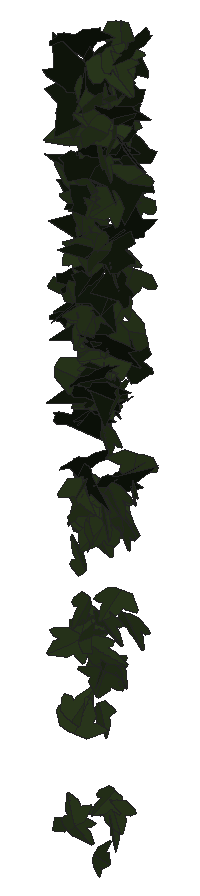
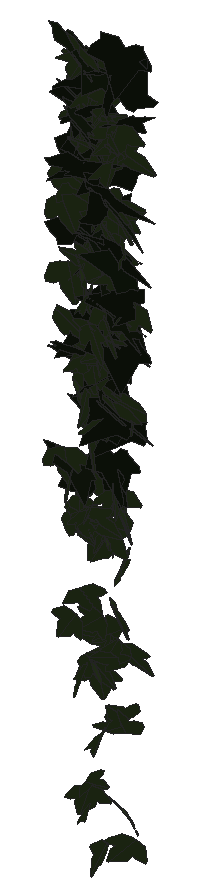
# SketchUp Ruby script. Lengths in inches.
U = 1.inch
M = Sketchup.active_model
def pt(a) = Geom::Point3d.new(a.map { |v| v * U })
def face(e, loops, mat)
  f = e.add_face(loops[0].map { |a| pt(a) })
  loops[1..].each { |l| e.add_face(l.map { |a| pt(a) }).erase! }
  f.material = f.back_material = mat if mat
  f
end
# faces: each face lists its corners as indices into pts; further lists are holes
def faces(e, pts, list, mat = nil) = list.each { |f| face(e, (f[0].is_a?(Array) ? f : [f]).map { |l| l.map { |i| pts[i] } }, mat) }
# xy, xz, yz: faces in a plane at the given z, y or x. An outline is a flat list of corners, or four numbers for a rectangle; further outlines are holes
def ring(l) = l.size == 4 ? [[l[0], l[1]], [l[2], l[1]], [l[2], l[3]], [l[0], l[3]]] : l.each_slice(2).to_a
def flat(e, list, mat, &to3) = list.each { |f| face(e, (f[0].is_a?(Array) ? f : [f]).map { |l| ring(l).map { |u, v| to3.(u, v) } }, mat) }
def xy(e, z, list, mat = nil) = flat(e, list, mat) { |x, y| [x, y, z] }
def xz(e, y, list, mat = nil) = flat(e, list, mat) { |x, z| [x, y, z] }
def yz(e, x, list, mat = nil) = flat(e, list, mat) { |y, z| [x, y, z] }
def lines(e, pts, list) = list.each { |a, b| e.add_line(pt(pts[a]), pt(pts[b])) }
# prism: a flat outline (further loops are holes) pulled along v
def prism(e, loops, v, mat = nil)
  f = face(e, loops, mat); d = Geom::Vector3d.new(v.map { |x| x * U })
  f.pushpull(f.normal.samedirection?(d) ? d.length : -d.length)
end
def box(e, o, s, mat = nil) = prism(e, [[o, [o[0] + s[0], o[1], o[2]], [o[0] + s[0], o[1] + s[1], o[2]], [o[0], o[1] + s[1], o[2]]]], [0, 0, s[2]], mat)
def at(x, y, z, deg = 0) = Geom::Transformation.translation(pt([x, y, z])) * Geom::Transformation.rotation(ORIGIN, Z_AXIS, deg.degrees)
def axes(o, x, y, z) = Geom::Transformation.new([*x, 0, *y, 0, *z, 0, *pt(o).to_a, 1])
def part(name) = M.definitions.add(name)
# library, detail: a bought-in or finely detailed component or shape, given as its bounding box
def library(name, o, s) = part(name).tap { |d| box(d.entities, o, s) }
def detail(e, o, s) = box(e.add_group.entities, o, s)
def put(e, d, t, mat = nil) = e.add_instance(d, t).tap { |i| i.material = mat if mat }
def group(e, t, mat = nil) = e.add_group.tap { |g| g.transformation = t; g.material = mat if mat }.entities
root = M.entities
M.materials.add("1026 AP 7946 SUNNY SIDE UP").color = [254, 231, 186]
M.materials.add("efeu1").color = [18, 25, 13]
M.materials.add("efeu2").color = [43, 57, 29]
c1 = part("ivyleaf_9")
p = [[1.54,2.16,1.25],[1.36,2.04,1.19],[-0.21,0.99,0.68],[-0.71,1.11,0.82],[-0.85,0.86,0.67],[-0.8,0.17,0.21],
  [-0.9,-0.01,0.1],[-0.67,-0.16,-0.02],[-0.08,-0.08,-0.05],[-0.03,-0.6,-0.4],[0.65,-0.88,-0.66],[0.83,-0.6,-0.49],
  [1.29,-0.42,-0.43],[1.8125,-0.07,-0.26],[1.21,0.44,0.15]]
faces(c1.entities,p,[[0,1,2,3,4,5,6,7,8,9,10,11,12,13,14]],"efeu1")
c2 = part("ivyleaf_10")
p = [[0,0.5,-0.03],[-0.0625,2.02,-0.43],[-0.19,2.01,-0.46],[-0.54,1.05,-0.29],[-0.52,0.625,-0.18],[-0.83,0.76,-0.28],
  [-1.16,0.64,-0.33],[-1.15,0.33,-0.24],[-0.77,-0.39,0.02],[-0.3,-0.51,0.16],[0.04,-0.48,0.23],[-0.02,2.01,-0.4375],
  [-0.06,2.01,-0.43],[0.04,-0.49,0.23],[0.67,-0.49,0.14],[1.38,0.36,-0.2],[1.375,0.51,-0.24],[0.81,0.65,-0.19],
  [0.62,0.59,-0.15],[0.6,1.09,-0.28],[0.5,1.23,-0.31]]
faces(c2.entities,p,[[0,1,2,3,4,5,6,7,8,9,10],[11,12,0,13,14,15,16,17,18,19,20]],"efeu2")
put(root,c1,axes([144.33,212.75,264.91],[-0.14477,0.20271,0.14343],[-0.09763,0.12342,-0.22859],[-0.3731,-0.11095,0.00416]),"1026 AP 7946 SUNNY SIDE UP")
put(root,c2,axes([144.375,212.71,265.98],[-0.19313,-0.02932,0.23995],[-0.32391,-0.11299,-0.12713],[0.17757,-0.238,0.02907]),"1026 AP 7946 SUNNY SIDE UP")
put(root,c2,axes([144.0625,212.68,263.17],[-0.37059,0.02772,-0.05912],[0.08531,-0.02917,-0.24359],[-0.05298,-0.24085,0.02125]),"1026 AP 7946 SUNNY SIDE UP")
put(root,c1,axes([144.14,212.86,262.6],[0.23847,0.17879,-0.10822],[-0.08985,-0.09038,-0.24165],[-0.31429,0.1615,-0.01303]),"1026 AP 7946 SUNNY SIDE UP")
put(root,c2,axes([144.39,212.74,264.93],[-0.15157,0.01941,-0.24619],[-0.33509,0.11135,0.09848],[0.17314,0.2325,-0.02493]),"1026 AP 7946 SUNNY SIDE UP")
put(root,c2,axes([143.85,212.85,261.51],[-0.01401,-0.04206,-0.23299],[0.32856,-0.09558,0.00928],[-0.15039,-0.2049,0.04199]),"1026 AP 7946 SUNNY SIDE UP")
put(root,c2,axes([144.24,212.6,256.93],[0.27563,-0.04144,-0.12893],[-0.20017,-0.00058,-0.18384],[0.05252,0.21525,-0.02401]),"1026 AP 7946 SUNNY SIDE UP")
put(root,c1,axes([144.43,212.85,264.24],[-0.08439,-0.01917,-0.25421],[-0.38224,-0.04278,0.05767],[-0.07224,0.24877,-0.00816]),"1026 AP 7946 SUNNY SIDE UP")
put(root,c2,axes([144.13,212.96,261.5],[0.36599,-0.07417,-0.01921],[-0.03604,-0.01206,-0.25102],[0.11456,0.23316,-0.0176]),"1026 AP 7946 SUNNY SIDE UP")
put(root,c2,axes([144.04,212.76,253.56],[-0.25435,-0.06715,-0.11637],[0.17582,0.02264,-0.17929],[0.10757,-0.19578,0.01789]),"1026 AP 7946 SUNNY SIDE UP")
put(root,c1,axes([144.47,212.96,265.19],[-0.2155,0.09765,0.19048],[-0.26082,0.08275,-0.17171],[-0.19892,-0.21428,0.01879]),"1026 AP 7946 SUNNY SIDE UP")
put(root,c1,axes([144.32,212.625,263.04],[-0.13864,0.24377,-0.07114],[0.03024,-0.06794,-0.2674],[-0.39784,-0.09012,0.00447]),"1026 AP 7946 SUNNY SIDE UP")
put(root,c1,axes([144.4,212.91,261.39],[-0.33839,0.1175,-0.00233],[-0.02931,-0.04016,-0.2487],[-0.18248,-0.21145,0.04428]),"1026 AP 7946 SUNNY SIDE UP")
put(root,c2,axes([144.27,212.79,264.34],[-0.28714,0.16387,0.07867],[-0.11276,0.03256,-0.2515],[-0.26028,-0.19488,0.02216]),"1026 AP 7946 SUNNY SIDE UP")
put(root,c2,axes([144.09,212.92,257],[-0.00415,-0.03981,0.2256],[0.07202,0.21445,0.04194],[-0.34285,0.04553,0.00608]),"1026 AP 7946 SUNNY SIDE UP")
put(root,c2,axes([144.19,212.77,259.43],[0.19238,-0.20792,0.03988],[0.02835,-0.03567,-0.24873],[0.33169,0.12365,-0.00187]),"1026 AP 7946 SUNNY SIDE UP")
put(root,c1,axes([144.23,212.82,266.53],[-0.2298,-0.19843,0.07366],[-0.04979,-0.06675,-0.25389],[0.3285,-0.14892,0.01305]),"1026 AP 7946 SUNNY SIDE UP")
put(root,c1,axes([144.1,212.8,263.96],[-0.03082,0.24079,-0.10846],[-0.01214,0.10638,0.24951],[0.41392,0.02105,-0.00076]),"1026 AP 7946 SUNNY SIDE UP")
put(root,c2,axes([144.4,212.95,262.86],[-0.13157,0.10088,0.19212],[-0.26924,0.08507,-0.12645],[-0.19526,-0.18527,0.04491]),"1026 AP 7946 SUNNY SIDE UP")
put(root,c1,axes([144.34,212.64,266.91],[0.26982,0.00708,0.23695],[-0.34068,0.10148,0.16393],[-0.1217,-0.26838,0.06644]),"1026 AP 7946 SUNNY SIDE UP")
put(root,c2,axes([144.26,213.07,256.97],[0.20492,0.16475,0.0384],[-0.05162,-0.02028,0.21588],[0.26022,-0.13377,0.01258]),"1026 AP 7946 SUNNY SIDE UP")
put(root,c2,axes([144.37,212.45,253.84],[0.22327,0.01225,0.19043],[-0.23997,0.13963,0.11209],[-0.16494,-0.18657,0.09469]),"1026 AP 7946 SUNNY SIDE UP")
put(root,c1,axes([144.27,212.62,267.77],[0.2048,0.22781,-0.03824],[-0.01325,-0.03939,-0.27028],[-0.36302,0.12996,-0.01171]),"1026 AP 7946 SUNNY SIDE UP")
put(root,c2,axes([144.3,212.6875,258.3],[-0.11517,0.22606,0.01893],[0.0148,-0.01492,0.24468],[0.35617,0.07372,-0.00405]),"1026 AP 7946 SUNNY SIDE UP")
put(root,c2,axes([144.21,212.8,263.8],[0.18184,0.22084,-0.02643],[-0.00393,-0.02903,-0.25673],[-0.3498,0.11513,-0.01085]),"1026 AP 7946 SUNNY SIDE UP")
put(root,c2,axes([144.37,212.75,264.92],[0.24578,-0.1781,-0.11169],[-0.13273,0.06847,-0.24311],[0.29887,0.17686,-0.01612]),"1026 AP 7946 SUNNY SIDE UP")
put(root,c2,axes([144.27,212.83,266.39],[-0.30222,-0.16122,-0.05344],[0.08532,0.01425,-0.25723],[0.2518,-0.19833,0.02302]),"1026 AP 7946 SUNNY SIDE UP")
put(root,c2,axes([144.26,212.73,262.96],[-0.05102,0.23097,-0.05017],[0.0007,-0.05042,-0.24048],[-0.37159,-0.03181,0.00644]),"1026 AP 7946 SUNNY SIDE UP")
put(root,c1,axes([144.08,212.68,263.23],[0.13025,0.04303,0.23122],[0.32615,0.08543,-0.09534],[-0.14994,0.22322,-0.00654]),"1026 AP 7946 SUNNY SIDE UP")
put(root,c2,axes([144.36,212.72,259.8],[0.0357,-0.17419,-0.1269],[-0.02349,0.12128,-0.18026],[0.33375,0.02717,0.00089]),"1026 AP 7946 SUNNY SIDE UP")
put(root,c2,axes([144.4,212.66,264.78],[-0.41571,0.05676,0.02734],[-0.05629,-0.04404,-0.27396],[-0.0806,-0.262,0.05033]),"1026 AP 7946 SUNNY SIDE UP")
put(root,c1,axes([144.2,212.94,261.35],[0.37383,0.05233,-0.01146],[-0.00995,-0.02417,-0.24988],[-0.08363,0.23679,-0.02151]),"1026 AP 7946 SUNNY SIDE UP")
put(root,c2,axes([144.27,212.6875,266.25],[-0.05335,-0.09952,-0.25052],[0.16653,0.21859,-0.10636],[0.3772,-0.11058,0.01153]),"1026 AP 7946 SUNNY SIDE UP")
put(root,c2,axes([144.51,212.83,262.3125],[-0.2973,-0.04335,0.11487],[-0.15334,-0.0657,-0.19663],[0.10958,-0.20957,0.03649]),"1026 AP 7946 SUNNY SIDE UP")
put(root,c2,axes([144.3,212.54,255.67],[0.13496,0.13403,-0.17783],[0.12232,0.15544,0.16438],[0.32215,-0.11517,0.01208]),"1026 AP 7946 SUNNY SIDE UP")
put(root,c2,axes([144.33,212.89,265.77],[0.06463,0.24885,-0.03918],[-0.0057,-0.03938,-0.26005],[-0.39613,0.04117,-0.00265]),"1026 AP 7946 SUNNY SIDE UP")
put(root,c2,axes([144.39,212.67,257.62],[0.23585,-0.18361,0.0049],[-0.01176,-0.01358,-0.24388],[0.28862,0.14949,-0.01394]),"1026 AP 7946 SUNNY SIDE UP")
put(root,c1,axes([144.28,212.99,267.21],[-0.03085,-0.00589,-0.26698],[0.29887,-0.17699,-0.01172],[-0.27707,-0.19026,0.01709]),"1026 AP 7946 SUNNY SIDE UP")
put(root,c1,axes([144.63,212.81,262.64],[-0.36437,0.09913,0.00317],[-0.0419,-0.0561,-0.25199],[-0.15019,-0.22485,0.06262]),"1026 AP 7946 SUNNY SIDE UP")
put(root,c2,axes([144.33,212.71,259.72],[-0.22034,-0.1962,-0.05143],[0.17081,-0.02298,-0.22627],[0.26811,-0.1466,0.10188]),"1026 AP 7946 SUNNY SIDE UP")
put(root,c2,axes([144.17,212.84,262.44],[0.13109,0.09804,0.22994],[0.23989,0.16225,-0.13151],[-0.29795,0.17377,-0.00472]),"1026 AP 7946 SUNNY SIDE UP")
put(root,c2,axes([144.32,212.63,259.1],[-0.05236,-0.09457,0.20525],[0.07628,0.19397,0.10406],[-0.33906,0.05824,-0.00828]),"1026 AP 7946 SUNNY SIDE UP")
put(root,c2,axes([144.59,213.05,262.73],[-0.25829,0.08136,0.13215],[-0.20373,0.02229,-0.18603],[-0.12349,-0.20694,0.03051]),"1026 AP 7946 SUNNY SIDE UP")
put(root,c2,axes([144.33,212.56,255.46],[0.31857,0.08972,-0.07676],[0.09372,0.04989,0.22759],[0.15822,-0.2102,0.01974]),"1026 AP 7946 SUNNY SIDE UP")
put(root,c1,axes([144.32,212.5,261.03],[0.33928,0.14496,0.00846],[0.02036,-0.00603,-0.26753],[-0.22732,0.21581,-0.01133]),"1026 AP 7946 SUNNY SIDE UP")
put(root,c2,axes([144.39,213.1,255.53],[-0.01316,0.20261,-0.02141],[0.00196,-0.0219,-0.20903],[-0.32043,-0.00845,-0.0004]),"1026 AP 7946 SUNNY SIDE UP")
put(root,c2,axes([144.39,212.67,262.76],[0.3307,-0.15598,0.04798],[0.04074,-0.04451,-0.26922],[0.25311,0.21096,-0.01936]),"1026 AP 7946 SUNNY SIDE UP")
put(root,c1,axes([144.52,212.57,260.3125],[0.06261,0.24305,-0.0547],[-0.00914,-0.05425,-0.25403],[-0.39155,0.04013,-0.00282]),"1026 AP 7946 SUNNY SIDE UP")
put(root,c2,axes([144.6,212.97,261.03],[-0.02991,-0.04333,-0.24145],[-0.24341,-0.17621,0.04552],[-0.28446,0.15533,-0.01356]),"1026 AP 7946 SUNNY SIDE UP")
put(root,c2,axes([144.69,212.75,266.26],[0.02495,-0.05643,-0.27895],[-0.26933,0.21055,-0.05437],[0.34086,0.17049,-0.02254]),"1026 AP 7946 SUNNY SIDE UP")
put(root,c2,axes([144.57,212.62,258.82],[0.1322,-0.01527,0.19052],[-0.1836,0.15357,0.06861],[-0.22696,-0.13312,0.05547]),"1026 AP 7946 SUNNY SIDE UP")
put(root,c2,axes([144.26,212.8,264.2],[0.107,-0.10147,-0.22658],[0.22321,-0.16766,0.12428],[-0.30758,-0.15697,0.01137]),"1026 AP 7946 SUNNY SIDE UP")
put(root,c1,axes([144.71,212.8,263.2],[-0.36056,0.11769,-0.01662],[-0.02493,-0.06645,-0.257],[-0.18527,-0.22011,0.06693]),"1026 AP 7946 SUNNY SIDE UP")
put(root,c2,axes([144.68,213,259.33],[-0.14537,-0.09107,0.19481],[-0.18722,-0.14809,-0.13394],[0.27266,-0.15024,0.01189]),"1026 AP 7946 SUNNY SIDE UP")
put(root,c2,axes([144.45,212.67,266.94],[0.05942,0.2528,0.13267],[0.01145,0.12757,-0.26236],[-0.44494,0.03705,0.01097]),"1026 AP 7946 SUNNY SIDE UP")
put(root,c2,axes([144.47,212.97,261.11],[0.08747,0.22265,-0.01549],[0.00043,-0.01687,-0.23648],[-0.35104,0.05546,-0.00415]),"1026 AP 7946 SUNNY SIDE UP")
put(root,c2,axes([144.66,212.84,261.53],[-0.30667,-0.044,0.08972],[-0.12042,-0.05246,-0.20371],[0.09564,-0.20715,0.03119]),"1026 AP 7946 SUNNY SIDE UP")
put(root,c2,axes([144.61,212.6875,264.05],[-0.38792,-0.09699,0.03935],[-0.0375,-0.04446,-0.27131],[0.15989,-0.24574,0.03185]),"1026 AP 7946 SUNNY SIDE UP")
put(root,c2,axes([144.49,212.8125,258.96],[-0.35345,-0.02324,-0.07557],[0.11806,-0.01858,-0.23149],[0.02554,-0.23568,0.0243]),"1026 AP 7946 SUNNY SIDE UP")
put(root,c2,axes([144.53,212.67,259.09],[-0.0119,0.17294,0.14778],[-0.04068,0.14092,-0.17682],[-0.34997,-0.02226,0.01553]),"1026 AP 7946 SUNNY SIDE UP")
put(root,c2,axes([144.59,212.62,262.92],[-0.22478,-0.20654,0.03436],[0.02173,-0.05102,-0.25577],[0.32856,-0.13793,0.04042]),"1026 AP 7946 SUNNY SIDE UP")
put(root,c1,axes([144.4,212.6875,265.61],[-0.04961,-0.10644,-0.23758],[0.0939,0.22214,-0.11304],[0.3873,-0.06749,-0.00302]),"1026 AP 7946 SUNNY SIDE UP")
put(root,c1,axes([144.55,212.73,264.73],[-0.2086,-0.08057,0.23088],[0.26903,0.14696,0.1593],[-0.26147,0.21549,-0.02029]),"1026 AP 7946 SUNNY SIDE UP")
put(root,c1,axes([144.28,212.72,259.92],[0.07231,-0.02626,-0.24968],[0.38222,-0.01166,0.04878],[-0.02581,-0.24627,0.02285]),"1026 AP 7946 SUNNY SIDE UP")
put(root,c2,axes([144.7,212.72,259.06],[-0.28946,-0.08571,0.12858],[-0.11548,-0.12209,-0.1979],[0.20891,-0.18623,0.06877]),"1026 AP 7946 SUNNY SIDE UP")
put(root,c2,axes([144.8,212.79,256.62],[-0.20578,0.00904,0.17501],[-0.26682,-0.02134,-0.13366],[0.01797,-0.21334,0.01952]),"1026 AP 7946 SUNNY SIDE UP")
put(root,c1,axes([144.63,212.86,267.42],[0.08908,0.17565,0.17823],[0.03686,0.17186,-0.18773],[-0.38481,0.05712,0.02328]),"1026 AP 7946 SUNNY SIDE UP")
put(root,c2,axes([144.57,212.48,257.1],[0.01372,-0.00271,0.21846],[-0.02879,0.21145,0.0048],[-0.33225,-0.01843,0.00861]),"1026 AP 7946 SUNNY SIDE UP")
put(root,c1,axes([144.45,212.63,260.96],[0.1173,0.22521,-0.046],[0.00866,0.04652,0.24449],[0.3613,-0.07423,0.00907]),"1026 AP 7946 SUNNY SIDE UP")
put(root,c1,axes([144.7,212.41,263.57],[0.06035,0.16785,0.20095],[0.00981,0.1956,-0.17437],[-0.40338,0.02987,0.02582]),"1026 AP 7946 SUNNY SIDE UP")
put(root,c2,axes([144.71,212.91,260.66],[0.10767,-0.13717,-0.19237],[-0.08453,0.17917,-0.1555],[0.35337,0.08466,0.02142]),"1026 AP 7946 SUNNY SIDE UP")
put(root,c1,axes([144.6875,212.45,261.91],[0.10404,0.23417,0.03538],[0.02419,0.02995,-0.25042],[-0.37106,0.06761,-0.0064]),"1026 AP 7946 SUNNY SIDE UP")
put(root,c2,axes([144.6875,212.65,253.19],[-0.00183,0.13418,0.17768],[-0.09897,0.16419,-0.13165],[-0.32805,-0.05028,0.03873]),"1026 AP 7946 SUNNY SIDE UP")
put(root,c2,axes([144.76,212.71,256.4375],[-0.31812,-0.04695,0.0604],[-0.08202,-0.03446,-0.21307],[0.08544,-0.20788,0.02037]),"1026 AP 7946 SUNNY SIDE UP")
put(root,c2,axes([144.76,212.83,262.0625],[-0.34763,-0.10097,0.04162],[-0.04734,-0.03246,-0.24998],[0.16467,-0.22249,0.01599]),"1026 AP 7946 SUNNY SIDE UP")
put(root,c2,axes([144.8,212.88,262.65],[-0.35581,0.09621,0.06382],[-0.13885,-0.06119,-0.23683],[-0.1137,-0.22634,0.08949]),"1026 AP 7946 SUNNY SIDE UP")
put(root,c1,axes([144.55,212.66,263.47],[0.08497,-0.24048,-0.11086],[-0.04894,0.10185,-0.25321],[0.41049,0.06192,-0.00724]),"1026 AP 7946 SUNNY SIDE UP")
put(root,c2,axes([144.42,212.84,265.86],[0.22352,-0.00537,-0.21978],[0.32186,0.0758,0.13901],[0.09473,-0.24487,0.04628]),"1026 AP 7946 SUNNY SIDE UP")
put(root,c2,axes([144.52,212.93,262.13],[-0.12005,0.08689,0.22645],[0.26623,-0.14033,0.11718],[0.25828,0.18503,-0.01553]),"1026 AP 7946 SUNNY SIDE UP")
put(root,c2,axes([144.76,212.96,259.38],[0.20692,0.09636,-0.13807],[-0.151,-0.09558,-0.1678],[-0.21197,0.16215,-0.01524]),"1026 AP 7946 SUNNY SIDE UP")
put(root,c2,axes([144.72,212.99,261.48],[0.00146,-0.15862,-0.18166],[0.01994,0.17522,-0.16211],[0.37136,-0.00879,0.00942]),"1026 AP 7946 SUNNY SIDE UP")
put(root,c2,axes([144.91,212.79,262.2],[0.23961,-0.02087,-0.19584],[-0.30015,-0.00448,-0.15725],[0.01502,0.24351,-0.01824]),"1026 AP 7946 SUNNY SIDE UP")
put(root,c2,axes([144.68,212.84,256.65],[0.12382,-0.16277,0.13061],[0.08202,-0.11661,-0.18693],[0.31481,0.0944,-0.00267]),"1026 AP 7946 SUNNY SIDE UP")
put(root,c1,axes([144.75,212.69,265.9],[0.21195,0.20119,-0.05971],[-0.03883,-0.05455,-0.24961],[-0.32743,0.1367,-0.00905]),"1026 AP 7946 SUNNY SIDE UP")
put(root,c2,axes([144.78,212.7,260.88],[-0.31311,0.12009,0.01714],[-0.03707,-0.0083,-0.23878],[-0.18684,-0.19959,0.01865]),"1026 AP 7946 SUNNY SIDE UP")
put(root,c1,axes([144.68,212.49,261.65],[0.29462,0.1554,0.00443],[0.0193,-0.00946,-0.25035],[-0.24364,0.18716,-0.01448]),"1026 AP 7946 SUNNY SIDE UP")
put(root,c2,axes([144.72,213.04,259.42],[0.0507,0.20023,-0.01472],[-0.00082,-0.01554,-0.20902],[-0.31578,0.03219,-0.00182]),"1026 AP 7946 SUNNY SIDE UP")
put(root,c1,axes([144.68,212.82,261.67],[-0.06606,-0.24676,0.02127],[-0.00202,-0.02214,-0.25798],[0.38954,-0.04196,0.00227]),"1026 AP 7946 SUNNY SIDE UP")
put(root,c2,axes([144.72,212.98,263.32],[-0.04693,0.22299,-0.06428],[0.01094,-0.0633,-0.23213],[-0.36447,-0.03061,0.00131]),"1026 AP 7946 SUNNY SIDE UP")
put(root,c1,axes([145.07,212.76,264.15],[-0.34776,0.04546,0.13039],[-0.20692,-0.02534,-0.22813],[-0.04169,-0.25342,0.04465]),"1026 AP 7946 SUNNY SIDE UP")
put(root,c1,axes([144.875,213.1875,266.71],[-0.29811,0.08727,-0.12493],[0.13729,-0.09523,-0.21091],[-0.19142,-0.20421,0.04329]),"1026 AP 7946 SUNNY SIDE UP")
put(root,c2,axes([144.88,212.86,263.57],[0.11705,-0.05738,0.2283],[-0.20968,0.17897,0.09479],[-0.29319,-0.1509,0.02336]),"1026 AP 7946 SUNNY SIDE UP")
put(root,c2,axes([144.75,212.69,265.875],[-0.07605,0.25242,0.01205],[-0.01809,0.00824,-0.26454],[-0.39683,-0.04875,0.00975]),"1026 AP 7946 SUNNY SIDE UP")
put(root,c1,axes([145.07,213.1,265.57],[-0.11652,0.05154,0.23473],[-0.36682,-0.01239,-0.07544],[-0.00611,-0.239,0.05306]),"1026 AP 7946 SUNNY SIDE UP")
put(root,c2,axes([145.01,212.68,266.24],[0.08857,0.13571,0.2169],[-0.26261,-0.13947,0.13834],[0.29217,-0.1665,0.05859]),"1026 AP 7946 SUNNY SIDE UP")
put(root,c2,axes([144.76,213,262.2],[0.1267,0.2035,-0.08945],[-0.0371,-0.08522,-0.2258],[-0.34663,0.0835,-0.00853]),"1026 AP 7946 SUNNY SIDE UP")
put(root,c1,axes([144.84,213.1,266.625],[-0.19905,-0.18384,0.10924],[-0.07273,-0.09785,-0.22995],[0.32653,-0.13386,0.01538]),"1026 AP 7946 SUNNY SIDE UP")
put(root,c2,axes([144.76,212.74,259.39],[-0.05418,0.20717,-0.06839],[0.01281,-0.06713,-0.21673],[-0.3424,-0.03529,0.00271]),"1026 AP 7946 SUNNY SIDE UP")
put(root,c2,axes([144.69,212.79,257.43],[-0.24631,0.07121,-0.1193],[0.15293,-0.06562,-0.17687],[-0.15013,-0.18368,0.01557]),"1026 AP 7946 SUNNY SIDE UP")
put(root,c2,axes([144.74,212.44,266.65],[0.03585,-0.08535,0.25674],[0.03274,0.25043,0.08769],[-0.41364,0.01243,0.02919]),"1026 AP 7946 SUNNY SIDE UP")
put(root,c1,axes([144.96,212.52,264.34],[-0.02829,0.24396,0.06777],[-0.01735,0.06374,-0.25156],[-0.39637,-0.0202,0.00617]),"1026 AP 7946 SUNNY SIDE UP")
put(root,c2,axes([144.83,212.96,256.52],[-0.09485,0.19084,0.07841],[-0.04972,0.06861,-0.20559],[-0.31858,-0.06753,0.00874]),"1026 AP 7946 SUNNY SIDE UP")
put(root,c1,axes([144.78,213.22,267.33],[-0.13375,-0.2255,0.02518],[-0.0021,-0.02697,-0.2483],[0.35688,-0.08467,0.00797]),"1026 AP 7946 SUNNY SIDE UP")
put(root,c2,axes([145.04,212.75,259.37],[-0.22426,0.05194,0.17142],[-0.26628,0.00807,-0.15235],[-0.06306,-0.21878,0.03372]),"1026 AP 7946 SUNNY SIDE UP")
put(root,c2,axes([144.8,212.86,266.91],[0.04126,0.24022,-0.05775],[-0.01488,-0.05672,-0.24925],[-0.38807,0.02772,0.00342]),"1026 AP 7946 SUNNY SIDE UP")
put(root,c2,axes([145.08,212.93,259.16],[-0.14834,0.03081,0.19129],[-0.29263,0.01446,-0.09989],[-0.0424,-0.20762,0.02018]),"1026 AP 7946 SUNNY SIDE UP")
put(root,c2,axes([144.72,213.12,267.81],[0.31524,-0.08948,0.11834],[0.14865,-0.0698,-0.22541],[0.17496,0.22053,-0.0217]),"1026 AP 7946 SUNNY SIDE UP")
put(root,c2,axes([144.9,212.85,257.85],[0.21415,0.14732,-0.09938],[-0.13292,-0.05347,-0.20562],[-0.24372,0.15861,0.02482]),"1026 AP 7946 SUNNY SIDE UP")
put(root,c2,axes([144.84,212.42,264.22],[-0.05029,-0.12366,-0.25568],[0.098,0.23951,-0.13018],[0.42384,-0.07006,-0.00024]),"1026 AP 7946 SUNNY SIDE UP")
put(root,c2,axes([144.77,212.46,266.36],[-0.12122,-0.13337,-0.21174],[0.20308,0.16005,-0.15655],[0.32622,-0.1492,0.01877]),"1026 AP 7946 SUNNY SIDE UP")
put(root,c2,axes([144.91,212.69,254.35],[0.09612,0.09994,-0.17389],[-0.10664,-0.15576,-0.12082],[-0.29025,0.09032,-0.0132]),"1026 AP 7946 SUNNY SIDE UP")
put(root,c2,axes([144.82,212.75,266.41],[-0.38245,-0.09777,-0.09221],[0.15041,-0.00164,-0.26761],[0.14343,-0.25897,0.03477]),"1026 AP 7946 SUNNY SIDE UP")
put(root,c2,axes([144.65,212.59,256.98],[-0.09939,-0.02423,-0.20531],[0.30811,-0.05227,-0.05783],[-0.0677,-0.2023,0.03825]),"1026 AP 7946 SUNNY SIDE UP")
put(root,c2,axes([144.63,213,263.95],[-0.0555,-0.0089,-0.24173],[0.3253,-0.11331,-0.0283],[-0.17449,-0.20843,0.02412]),"1026 AP 7946 SUNNY SIDE UP")
put(root,c2,axes([145.02,212.58,265.07],[0.27436,-0.14298,-0.1203],[-0.1633,0.05547,-0.23112],[0.239,0.20203,-0.01981]),"1026 AP 7946 SUNNY SIDE UP")
put(root,c1,axes([145.12,212.66,266.14],[-0.08758,0.19338,0.14778],[-0.09767,0.12956,-0.20559],[-0.36472,-0.08113,0.01957]),"1026 AP 7946 SUNNY SIDE UP")
put(root,c2,axes([144.98,212.87,265.08],[-0.28509,-0.17073,0.00061],[0.01748,-0.01408,-0.25598],[0.2679,-0.18077,0.01735]),"1026 AP 7946 SUNNY SIDE UP")
put(root,c2,axes([144.92,212.74,263.8],[-0.1124,0.22619,0.00085],[-0.00838,-0.00217,-0.24432],[-0.35556,-0.07145,0.00549]),"1026 AP 7946 SUNNY SIDE UP")
put(root,c2,axes([144.91,212.6875,259.86],[-0.3207,0.07293,-0.06601],[0.08034,-0.04723,-0.22179],[-0.1303,-0.20863,0.02571]),"1026 AP 7946 SUNNY SIDE UP")
put(root,c1,axes([144.76,212.54,262.52],[0.41495,0.05139,0.02907],[0.0435,0.00402,-0.27694],[-0.08103,0.26534,0.00018]),"1026 AP 7946 SUNNY SIDE UP")
put(root,c1,axes([145.1,212.8125,260.14],[-0.00241,0.23992,0.05677],[-0.04443,0.05322,-0.24526],[-0.38404,-0.00766,0.02802]),"1026 AP 7946 SUNNY SIDE UP")
put(root,c1,axes([145.23,212.78,266.77],[-0.24954,0.17203,0.08316],[-0.11068,0.04311,-0.23986],[-0.27684,-0.1723,0.02094]),"1026 AP 7946 SUNNY SIDE UP")
put(root,c2,axes([145,212.63,266.2],[-0.0068,-0.11488,-0.22795],[0.01179,0.22049,-0.11715],[0.39094,-0.00865,-0.00043]),"1026 AP 7946 SUNNY SIDE UP")
put(root,c2,axes([144.9375,212.7,254.17],[-0.25386,-0.13753,-0.03412],[0.10871,-0.03409,-0.20646],[0.19374,-0.16109,0.07114]),"1026 AP 7946 SUNNY SIDE UP")
put(root,c2,axes([144.77,212.72,267.4],[0.26915,0.13,0.1587],[0.20975,0.07717,-0.22039],[-0.23643,0.21645,-0.01485]),"1026 AP 7946 SUNNY SIDE UP")
put(root,c2,axes([144.89,212.84,267.55],[0.15756,0.22175,0.06459],[0.05093,0.05275,-0.25026],[-0.35822,0.10504,-0.00717]),"1026 AP 7946 SUNNY SIDE UP")
put(root,c2,axes([144.95,212.6875,253.89],[-0.04337,0.18787,-0.07552],[0.01379,-0.07388,-0.19604],[-0.31741,-0.02888,0.0018]),"1026 AP 7946 SUNNY SIDE UP")
put(root,c2,axes([145.11,212.97,263.64],[-0.36143,-0.09561,0.05211],[-0.06484,-0.03375,-0.2562],[0.15767,-0.23304,0.0141]),"1026 AP 7946 SUNNY SIDE UP")
put(root,c2,axes([144.99,212.87,261.61],[0.1219,-0.17564,0.14309],[0.06524,-0.13424,-0.19811],[0.34699,0.08694,-0.01302]),"1026 AP 7946 SUNNY SIDE UP")
put(root,c1,axes([144.99,212.57,266.7],[0.29385,0.16466,-0.05165],[-0.04413,-0.04526,-0.25639],[-0.26747,0.18837,-0.01444]),"1026 AP 7946 SUNNY SIDE UP")
put(root,c1,axes([145.07,212.78,263.53],[-0.1395,-0.08678,0.21358],[-0.13155,-0.19468,-0.12168],[0.32878,-0.11471,0.04194]),"1026 AP 7946 SUNNY SIDE UP")
put(root,c1,axes([145.29,212.93,262.16],[-0.3385,0.03308,0.10746],[-0.1688,-0.02132,-0.2218],[-0.0319,-0.23818,0.03335]),"1026 AP 7946 SUNNY SIDE UP")
put(root,c2,axes([145.03,212.78,259.26],[-0.27168,0.13449,-0.01927],[0.00909,-0.02419,-0.22514],[-0.21349,-0.17218,0.01494]),"1026 AP 7946 SUNNY SIDE UP")
put(root,c2,axes([145.13,213.07,264.89],[-0.2562,-0.15841,0.06871],[-0.055,-0.06067,-0.2337],[0.26517,-0.16564,0.01791]),"1026 AP 7946 SUNNY SIDE UP")
put(root,c2,axes([145.2,212.96,265.41],[-0.20848,-0.10913,0.17882],[-0.1557,-0.14775,-0.17386],[0.28325,-0.16154,0.03605]),"1026 AP 7946 SUNNY SIDE UP")
put(root,c1,axes([144.99,212.92,264.34],[0.23079,0.16363,0.14252],[-0.20016,-0.06694,0.22179],[0.26986,-0.18959,0.04262]),"1026 AP 7946 SUNNY SIDE UP")
put(root,c2,axes([145.08,212.99,259.96],[-0.17091,0.1968,0.02458],[-0.05707,0.00572,-0.22966],[-0.30624,-0.1109,0.02908]),"1026 AP 7946 SUNNY SIDE UP")
put(root,c1,axes([145.26,212.83,267.78],[-0.12373,0.23089,0.07192],[-0.06993,0.0569,-0.24985],[-0.37217,-0.08745,0.02304]),"1026 AP 7946 SUNNY SIDE UP")
put(root,c2,axes([145.32,212.88,262.7],[-0.11522,0.07223,0.212],[-0.33863,0.00771,-0.0819],[-0.05016,-0.21792,0.06595]),"1026 AP 7946 SUNNY SIDE UP")
put(root,c1,axes([144.9375,212.93,265.85],[0.32943,-0.15965,-0.04089],[0.06841,-0.0067,0.27047],[-0.24912,-0.21296,0.0202]),"1026 AP 7946 SUNNY SIDE UP")
put(root,c1,axes([144.99,212.9375,265.44],[-0.1485,-0.2444,-0.04232],[0.03822,0.03313,-0.26951],[0.38745,-0.09694,0.01036]),"1026 AP 7946 SUNNY SIDE UP")
put(root,c1,axes([144.875,212.71,259.88],[0.22539,0.20074,-0.03933],[0.00424,0.04615,0.25314],[0.32161,-0.14129,0.02423]),"1026 AP 7946 SUNNY SIDE UP")
put(root,c2,axes([145.03,213.01,257.4],[-0.29116,0.08744,-0.07346],[0.0877,-0.04929,-0.21028],[-0.15479,-0.19239,0.01905]),"1026 AP 7946 SUNNY SIDE UP")
put(root,c2,axes([145.15,213.01,260.32],[-0.30454,-0.1243,0.0366],[-0.01255,-0.05361,-0.23373],[0.2032,-0.1896,0.04042]),"1026 AP 7946 SUNNY SIDE UP")
put(root,c2,axes([145.11,212.74,263.26],[0.2806,-0.14858,-0.00001],[-0.01601,-0.01353,-0.23867],[0.23309,0.17794,-0.01638]),"1026 AP 7946 SUNNY SIDE UP")
